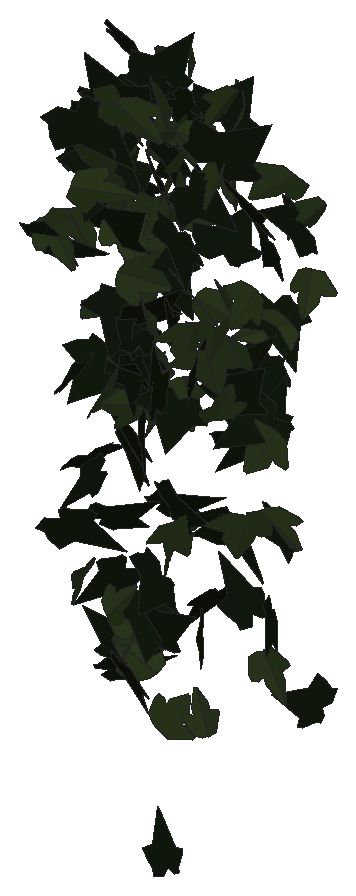
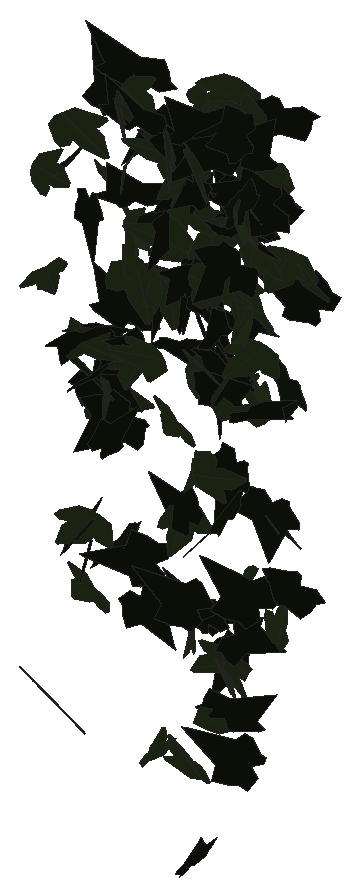
# SketchUp Ruby script. Lengths in inches.
U = 1.inch
M = Sketchup.active_model
def pt(a) = Geom::Point3d.new(a.map { |v| v * U })
def face(e, loops, mat)
  f = e.add_face(loops[0].map { |a| pt(a) })
  loops[1..].each { |l| e.add_face(l.map { |a| pt(a) }).erase! }
  f.material = f.back_material = mat if mat
  f
end
# faces: each face lists its corners as indices into pts; further lists are holes
def faces(e, pts, list, mat = nil) = list.each { |f| face(e, (f[0].is_a?(Array) ? f : [f]).map { |l| l.map { |i| pts[i] } }, mat) }
# xy, xz, yz: faces in a plane at the given z, y or x. An outline is a flat list of corners, or four numbers for a rectangle; further outlines are holes
def ring(l) = l.size == 4 ? [[l[0], l[1]], [l[2], l[1]], [l[2], l[3]], [l[0], l[3]]] : l.each_slice(2).to_a
def flat(e, list, mat, &to3) = list.each { |f| face(e, (f[0].is_a?(Array) ? f : [f]).map { |l| ring(l).map { |u, v| to3.(u, v) } }, mat) }
def xy(e, z, list, mat = nil) = flat(e, list, mat) { |x, y| [x, y, z] }
def xz(e, y, list, mat = nil) = flat(e, list, mat) { |x, z| [x, y, z] }
def yz(e, x, list, mat = nil) = flat(e, list, mat) { |y, z| [x, y, z] }
def lines(e, pts, list) = list.each { |a, b| e.add_line(pt(pts[a]), pt(pts[b])) }
# prism: a flat outline (further loops are holes) pulled along v
def prism(e, loops, v, mat = nil)
  f = face(e, loops, mat); d = Geom::Vector3d.new(v.map { |x| x * U })
  f.pushpull(f.normal.samedirection?(d) ? d.length : -d.length)
end
def box(e, o, s, mat = nil) = prism(e, [[o, [o[0] + s[0], o[1], o[2]], [o[0] + s[0], o[1] + s[1], o[2]], [o[0], o[1] + s[1], o[2]]]], [0, 0, s[2]], mat)
def at(x, y, z, deg = 0) = Geom::Transformation.translation(pt([x, y, z])) * Geom::Transformation.rotation(ORIGIN, Z_AXIS, deg.degrees)
def axes(o, x, y, z) = Geom::Transformation.new([*x, 0, *y, 0, *z, 0, *pt(o).to_a, 1])
def part(name) = M.definitions.add(name)
# library, detail: a bought-in or finely detailed component or shape, given as its bounding box
def library(name, o, s) = part(name).tap { |d| box(d.entities, o, s) }
def detail(e, o, s) = box(e.add_group.entities, o, s)
def put(e, d, t, mat = nil) = e.add_instance(d, t).tap { |i| i.material = mat if mat }
def group(e, t, mat = nil) = e.add_group.tap { |g| g.transformation = t; g.material = mat if mat }.entities
root = M.entities
M.materials.add("1026 AP 7946 SUNNY SIDE UP").color = [254, 231, 186]
M.materials.add("efeu1").color = [18, 25, 13]
M.materials.add("efeu2").color = [43, 57, 29]
c1 = part("ivyleaf_9")
p = [[1.54,2.16,1.25],[1.36,2.04,1.19],[-0.21,0.99,0.68],[-0.71,1.11,0.82],[-0.85,0.86,0.67],[-0.8,0.17,0.21],
  [-0.9,-0.01,0.1],[-0.67,-0.16,-0.02],[-0.08,-0.08,-0.05],[-0.03,-0.6,-0.4],[0.65,-0.88,-0.66],[0.83,-0.6,-0.49],
  [1.29,-0.42,-0.43],[1.8125,-0.07,-0.26],[1.21,0.44,0.15]]
faces(c1.entities,p,[[0,1,2,3,4,5,6,7,8,9,10,11,12,13,14]],"efeu1")
c2 = part("ivyleaf_10")
p = [[0,0.5,-0.03],[-0.0625,2.02,-0.43],[-0.19,2.01,-0.46],[-0.54,1.05,-0.29],[-0.52,0.625,-0.18],[-0.83,0.76,-0.28],
  [-1.16,0.64,-0.33],[-1.15,0.33,-0.24],[-0.77,-0.39,0.02],[-0.3,-0.51,0.16],[0.04,-0.48,0.23],[-0.02,2.01,-0.4375],
  [-0.06,2.01,-0.43],[0.04,-0.49,0.23],[0.67,-0.49,0.14],[1.38,0.36,-0.2],[1.375,0.51,-0.24],[0.81,0.65,-0.19],
  [0.62,0.59,-0.15],[0.6,1.09,-0.28],[0.5,1.23,-0.31]]
faces(c2.entities,p,[[0,1,2,3,4,5,6,7,8,9,10],[11,12,0,13,14,15,16,17,18,19,20]],"efeu2")
put(root,c1,axes([125.78,210.73,264.48],[0.12054,-0.07368,0.29819],[0.41686,-0.12179,-0.10483],[0.21772,0.27399,0.03562]),"1026 AP 7946 SUNNY SIDE UP")
put(root,c2,axes([125.89,211.97,264.9],[0.21507,-0.0579,0.27799],[0.37543,-0.12696,-0.1533],[0.21867,0.27492,-0.01023]),"1026 AP 7946 SUNNY SIDE UP")
put(root,c2,axes([125.91,210.6875,264.84],[0.3343,-0.00107,0.26157],[0.3907,-0.06728,-0.21503],[0.08218,0.32426,-0.04177]),"1026 AP 7946 SUNNY SIDE UP")
put(root,c1,axes([126.02,210.89,259.3],[0.02192,-0.00071,-0.30597],[0.18849,0.27204,0.00672],[0.42727,-0.11997,0.01273]),"1026 AP 7946 SUNNY SIDE UP")
put(root,c2,axes([126.32,211.97,266.5],[0.11014,-0.2742,0.11862],[0.03145,-0.11528,-0.29209],[0.46752,0.07235,-0.0083]),"1026 AP 7946 SUNNY SIDE UP")
put(root,c2,axes([126.66,212.47,261.83],[-0.1517,0.03049,-0.28411],[-0.41399,0.08267,0.10472],[0.13855,0.2804,0.00182]),"1026 AP 7946 SUNNY SIDE UP")
put(root,c2,axes([126.29,211.89,264.6],[-0.28844,0.25395,-0.1145],[0.07835,-0.10265,-0.32276],[-0.42971,-0.18918,0.018]),"1026 AP 7946 SUNNY SIDE UP")
put(root,c2,axes([126.35,210.76,265.17],[-0.42324,-0.12548,-0.09661],[0.15222,0.01154,-0.30441],[0.19279,-0.28457,0.02827]),"1026 AP 7946 SUNNY SIDE UP")
put(root,c2,axes([126.375,210.97,258.3125],[-0.02671,-0.17761,-0.27305],[-0.00878,-0.26421,0.18191],[-0.50029,0.01412,0.01138]),"1026 AP 7946 SUNNY SIDE UP")
put(root,c1,axes([126.51,210.95,260.67],[0.10897,0.30312,0.00846],[0.01022,0.00517,-0.32026],[-0.47663,0.06941,-0.00494]),"1026 AP 7946 SUNNY SIDE UP")
put(root,c2,axes([126.23,211.7,265.76],[0.4966,-0.0822,0.15346],[0.21456,-0.06688,-0.33539],[0.16088,0.34293,-0.02642]),"1026 AP 7946 SUNNY SIDE UP")
put(root,c1,axes([125.98,211.66,266.73],[0.19799,0.05636,-0.34035],[0.41951,0.19731,0.14045],[0.31977,-0.29374,0.02648]),"1026 AP 7946 SUNNY SIDE UP")
put(root,c1,axes([126.21,212.02,266.68],[0.15385,-0.20438,0.19255],[0.10869,-0.17521,-0.23423],[0.42299,0.11936,-0.00985]),"1026 AP 7946 SUNNY SIDE UP")
put(root,c2,axes([126.52,211.8,265.09],[-0.09459,-0.29834,-0.04622],[0.03148,0.03997,-0.31307],[0.47295,-0.06233,0.01159]),"1026 AP 7946 SUNNY SIDE UP")
put(root,c1,axes([126.39,211.0625,265.95],[-0.09339,0.0031,0.37339],[0.51727,0.15462,0.05508],[-0.23921,0.33313,-0.02667]),"1026 AP 7946 SUNNY SIDE UP")
put(root,c1,axes([126.33,211.59,259.15],[0.37331,0.18571,-0.05497],[0.03981,0.05558,0.30953],[0.30168,-0.23715,0.02718]),"1026 AP 7946 SUNNY SIDE UP")
put(root,c1,axes([126.28,211.96,267.99],[0.39241,-0.15583,0.11286],[0.12773,-0.07786,-0.30274],[0.27181,0.26156,-0.02067]),"1026 AP 7946 SUNNY SIDE UP")
put(root,c1,axes([126.86,211.67,265.96],[-0.47227,-0.05249,0.03408],[-0.04285,-0.03694,-0.31264],[0.08794,-0.29993,0.03071]),"1026 AP 7946 SUNNY SIDE UP")
put(root,c1,axes([126.77,210.16,262.53],[0.0099,0.23389,0.19022],[0.01171,0.18318,-0.23995],[-0.46712,0.00955,-0.00198]),"1026 AP 7946 SUNNY SIDE UP")
put(root,c1,axes([126.36,211.74,256.27],[0.27108,0.225,-0.11548],[0.08344,0.10187,0.29199],[0.38728,-0.17944,0.01792]),"1026 AP 7946 SUNNY SIDE UP")
put(root,c2,axes([126.39,211.65,266.43],[0.28057,-0.07256,0.24354],[0.34143,-0.09458,-0.19895],[0.18735,0.28102,-0.00214]),"1026 AP 7946 SUNNY SIDE UP")
put(root,c1,axes([126.92,211.57,256.87],[0.10544,0.03542,0.28985],[-0.44207,0.04453,0.06356],[-0.05584,-0.28559,0.04412]),"1026 AP 7946 SUNNY SIDE UP")
put(root,c1,axes([126.84,211.375,267.16],[0.25958,-0.00539,0.2712],[-0.39634,0.08672,0.16516],[-0.11986,-0.29841,0.0412]),"1026 AP 7946 SUNNY SIDE UP")
put(root,c1,axes([126.76,211.16,262.41],[-0.30762,-0.23846,0.12596],[-0.09814,-0.1084,-0.31779],[0.41079,-0.20447,0.01841]),"1026 AP 7946 SUNNY SIDE UP")
put(root,c1,axes([126.83,210.79,260.53],[-0.37257,0.13849,-0.12506],[0.14588,-0.08259,-0.28228],[-0.25109,-0.25348,0.02157]),"1026 AP 7946 SUNNY SIDE UP")
put(root,c1,axes([126.51,211.81,265.45],[0.45887,0.08022,0.00252],[0.01414,-0.02522,-0.31073],[-0.12539,0.29075,-0.0258]),"1026 AP 7946 SUNNY SIDE UP")
put(root,c1,axes([126.8,211.47,258.39],[-0.0435,0.00077,-0.31404],[0.10414,-0.29877,-0.00871],[-0.46789,-0.06657,0.02726]),"1026 AP 7946 SUNNY SIDE UP")
put(root,c2,axes([126.65,211.13,263.5],[-0.30292,-0.13622,-0.19501],[0.2703,0.0815,-0.24116],[0.24635,-0.25692,0.02482]),"1026 AP 7946 SUNNY SIDE UP")
put(root,c2,axes([127.2,211.83,264.95],[0.06842,-0.05078,-0.34035],[-0.48838,0.1162,-0.05992],[0.19302,0.31201,-0.03095]),"1026 AP 7946 SUNNY SIDE UP")
put(root,c2,axes([126.83,211.18,266.37],[0.07883,-0.13746,-0.3173],[0.10388,0.30859,-0.12933],[0.51893,-0.04089,0.07409]),"1026 AP 7946 SUNNY SIDE UP")
put(root,c2,axes([127,212.41,267.49],[0.22525,-0.20264,-0.1724],[-0.15575,0.13349,-0.25485],[0.38152,0.17413,-0.00225]),"1026 AP 7946 SUNNY SIDE UP")
put(root,c2,axes([126.93,212.12,261.76],[-0.02544,0.07802,0.28794],[-0.11575,0.26921,-0.08036],[-0.44066,-0.07522,0.00449]),"1026 AP 7946 SUNNY SIDE UP")
put(root,c1,axes([127.04,210.83,266.33],[-0.46572,-0.14302,-0.10495],[0.16211,0.0181,-0.33757],[0.22259,-0.31243,0.02627]),"1026 AP 7946 SUNNY SIDE UP")
put(root,c1,axes([126.88,211.78,267.5],[0.04828,-0.09551,-0.32711],[-0.00535,0.31823,-0.09726],[0.52053,0.01213,0.02934]),"1026 AP 7946 SUNNY SIDE UP")
put(root,c2,axes([127.21,211.58,256.69],[0.14116,0.22597,0.18684],[-0.1242,-0.1622,0.2493],[0.43704,-0.11908,0.0105]),"1026 AP 7946 SUNNY SIDE UP")
put(root,c1,axes([127.07,211.1875,261.32],[0.41086,-0.07086,-0.19853],[-0.30161,0.02519,-0.27791],[0.1135,0.32345,-0.01985]),"1026 AP 7946 SUNNY SIDE UP")
put(root,c1,axes([126.9,211.6,260.58],[0.05064,-0.2068,0.26901],[0.03786,-0.26139,-0.21688],[0.52384,0.03888,-0.01033]),"1026 AP 7946 SUNNY SIDE UP")
put(root,c1,axes([126.88,210.22,267.49],[-0.03588,-0.17005,-0.34523],[0.11108,0.32681,-0.1744],[0.57897,-0.07324,0.01207]),"1026 AP 7946 SUNNY SIDE UP")
put(root,c2,axes([127,210.63,266.33],[-0.47085,0.04161,0.15361],[0.22623,-0.04361,0.31045],[0.08885,0.33155,0.02356]),"1026 AP 7946 SUNNY SIDE UP")
put(root,c2,axes([127.28,211.27,257.68],[0.36603,-0.15599,-0.12256],[-0.1751,0.04526,-0.28748],[0.25294,0.25707,-0.02165]),"1026 AP 7946 SUNNY SIDE UP")
put(root,c2,axes([127.09,210.47,262.01],[0.08446,-0.3233,0.06138],[0.00964,0.0632,0.33759],[-0.51736,-0.0516,0.01631]),"1026 AP 7946 SUNNY SIDE UP")
put(root,c2,axes([127.25,212.04,258.61],[0.06787,-0.09362,-0.28402],[-0.02792,0.27681,-0.09828],[0.45617,0.03087,0.03624]),"1026 AP 7946 SUNNY SIDE UP")
put(root,c2,axes([127.22,211.33,257.59],[0.21684,-0.268,0.05727],[0.02122,-0.05722,-0.3105],[0.43034,0.13786,-0.01355]),"1026 AP 7946 SUNNY SIDE UP")
put(root,c1,axes([126.93,212.41,259.26],[0.33829,0.1653,-0.11727],[0.12075,0.08787,0.27918],[0.29249,-0.22746,0.02038]),"1026 AP 7946 SUNNY SIDE UP")
put(root,c2,axes([127.01,210.1875,266.18],[-0.09009,-0.0604,-0.33327],[0.41456,0.18752,-0.08316],[0.30881,-0.26935,0.01442]),"1026 AP 7946 SUNNY SIDE UP")
put(root,c2,axes([127,210.75,267.48],[-0.01121,0.00671,0.30978],[0.46548,0.05313,0.00632],[-0.08329,0.29601,-0.00637]),"1026 AP 7946 SUNNY SIDE UP")
put(root,c1,axes([127.36,210.85,263.82],[-0.38644,-0.14512,-0.11439],[0.17716,0.02443,-0.29181],[0.2252,-0.26823,0.03327]),"1026 AP 7946 SUNNY SIDE UP")
put(root,c2,axes([127.06,211.27,257.74],[0.24236,0.11274,0.24332],[0.33344,0.10558,-0.19439],[-0.23962,0.26094,-0.02441]),"1026 AP 7946 SUNNY SIDE UP")
put(root,c2,axes([127.45,212.43,267.64],[0.16323,-0.25345,-0.22182],[-0.05739,0.21402,-0.27827],[0.51829,0.10352,0.03904]),"1026 AP 7946 SUNNY SIDE UP")
put(root,c1,axes([127.26,211.75,267.58],[-0.19038,-0.06596,0.30627],[0.4351,0.1107,0.14187],[-0.20128,0.30168,0.01699]),"1026 AP 7946 SUNNY SIDE UP")
put(root,c2,axes([127.4375,211.56,264.52],[-0.05623,0.17635,0.30673],[0.07887,-0.29251,0.1836],[0.53701,0.06142,0.00515]),"1026 AP 7946 SUNNY SIDE UP")
put(root,c1,axes([127.26,210.57,265.31],[-0.17127,-0.01633,0.33508],[0.35546,-0.2508,0.06353],[0.36881,0.23413,0.09437]),"1026 AP 7946 SUNNY SIDE UP")
put(root,c1,axes([127.36,211.8,266.72],[0.4604,-0.08452,-0.03393],[-0.0618,-0.01967,-0.31258],[0.12824,0.29394,-0.02881]),"1026 AP 7946 SUNNY SIDE UP")
put(root,c2,axes([127.62,210.77,262.1],[-0.01517,0.12729,0.35315],[0.06368,-0.33971,0.12942],[0.57037,0.04131,-0.00506]),"1026 AP 7946 SUNNY SIDE UP")
put(root,c2,axes([127.45,210.7,265.375],[0.34569,0.22665,0.06981],[0.09908,0.03125,-0.32424],[-0.35793,0.22754,-0.02233]),"1026 AP 7946 SUNNY SIDE UP")
put(root,c2,axes([127.68,211.75,266.59],[0.04346,-0.00753,0.34432],[-0.12245,0.32604,0.01611],[-0.51129,-0.07872,0.02541]),"1026 AP 7946 SUNNY SIDE UP")
put(root,c2,axes([127.61,210.17,258.52],[0.05115,0.06951,-0.28899],[0.12448,0.26976,0.07979],[0.43767,-0.08485,0.01108]),"1026 AP 7946 SUNNY SIDE UP")
put(root,c1,axes([127.5,210.91,262.9],[-0.23222,-0.1177,-0.23213],[0.34677,0.06879,-0.18608],[0.19695,-0.25991,0.05393]),"1026 AP 7946 SUNNY SIDE UP")
put(root,c1,axes([127.53,210.9,262.33],[0.4637,-0.16133,0.01077],[0.00886,0.03388,0.34488],[-0.25415,-0.29317,0.03167]),"1026 AP 7946 SUNNY SIDE UP")
put(root,c1,axes([127.72,210.74,263.3],[-0.17694,-0.1372,0.29466],[0.25094,0.23875,0.18356],[-0.43236,0.19472,-0.01405]),"1026 AP 7946 SUNNY SIDE UP")
put(root,c2,axes([127.64,211.34,266.97],[-0.04865,-0.1505,-0.2973],[0.13835,0.27433,-0.15596],[0.49147,-0.09212,0.01448]),"1026 AP 7946 SUNNY SIDE UP")
put(root,c2,axes([127.66,211.42,266.58],[0.0542,-0.15422,0.28276],[-0.02385,0.27586,0.16274],[-0.49567,-0.03013,0.02309]),"1026 AP 7946 SUNNY SIDE UP")
put(root,c2,axes([127.5,211.6875,255.72],[0.4124,-0.11776,-0.11906],[0.18791,-0.01228,0.2939],[-0.17783,-0.28608,0.03444]),"1026 AP 7946 SUNNY SIDE UP")
put(root,c1,axes([127.64,210.4375,257.33],[0.40702,-0.08305,-0.14542],[-0.22483,0.01234,-0.27846],[0.12426,0.29436,-0.02749]),"1026 AP 7946 SUNNY SIDE UP")
put(root,c2,axes([127.74,211.19,267.79],[-0.31106,0.24008,-0.04286],[0.0176,-0.04633,-0.32004],[-0.38309,-0.19706,0.02009]),"1026 AP 7946 SUNNY SIDE UP")
put(root,c2,axes([127.61,210.49,267.73],[-0.40289,-0.10803,-0.2028],[0.3028,0.0461,-0.2849],[0.17995,-0.31944,0.02535]),"1026 AP 7946 SUNNY SIDE UP")
put(root,c1,axes([127.66,210.66,262.88],[-0.2204,-0.02321,-0.25732],[0.38941,-0.05748,-0.13808],[-0.06156,-0.28048,0.04787]),"1026 AP 7946 SUNNY SIDE UP")
put(root,c1,axes([127.8,211.6875,266.3125],[-0.0628,-0.12049,0.28843],[-0.13206,-0.26781,-0.13232],[0.46175,-0.09298,0.00139]),"1026 AP 7946 SUNNY SIDE UP")
put(root,c1,axes([127.83,210.97,258.29],[-0.32284,-0.19926,-0.11114],[0.14601,0.05714,-0.29353],[0.32408,-0.22425,0.02153]),"1026 AP 7946 SUNNY SIDE UP")
put(root,c1,axes([127.55,211.96,267.1875],[0.14626,-0.08622,-0.27948],[0.44658,0.03833,0.08815],[0.01589,-0.28375,0.09498]),"1026 AP 7946 SUNNY SIDE UP")
put(root,c1,axes([127.76,211.23,264.63],[-0.09831,-0.2241,-0.23097],[0.1208,0.20966,-0.2381],[0.48213,-0.09823,0.01256]),"1026 AP 7946 SUNNY SIDE UP")
put(root,c1,axes([128.01,211.69,265.62],[-0.00693,-0.01748,-0.30726],[-0.27088,0.24374,-0.01067],[0.38363,0.17178,-0.01309]),"1026 AP 7946 SUNNY SIDE UP")
put(root,c1,axes([127.8125,211.21,265.95],[-0.10562,0.00348,0.35669],[0.04243,-0.35155,0.00698],[0.54277,0.02816,0.06886]),"1026 AP 7946 SUNNY SIDE UP")
put(root,c1,axes([128.07,211.03,253.54],[-0.16897,-0.17454,0.21803],[0.14904,0.19081,0.21182],[-0.40607,0.14266,-0.01298]),"1026 AP 7946 SUNNY SIDE UP")
put(root,c2,axes([128.08,211.1875,265.79],[-0.09022,-0.28179,0.20872],[-0.04673,-0.20224,-0.29729],[0.5452,-0.06396,0.00906]),"1026 AP 7946 SUNNY SIDE UP")
put(root,c2,axes([128.03,210.55,264.17],[-0.17368,0.29491,0.08513],[-0.06866,0.06999,-0.32361],[-0.47595,-0.11771,0.01562]),"1026 AP 7946 SUNNY SIDE UP")
put(root,c1,axes([127.83,210.67,262.03],[-0.0862,0.00371,-0.35475],[0.48911,-0.14913,-0.05354],[-0.23243,-0.31521,0.0189]),"1026 AP 7946 SUNNY SIDE UP")
put(root,c1,axes([127.8125,210.63,263.85],[0.33208,0.23474,0.02834],[-0.05409,-0.00418,0.32443],[0.36744,-0.21277,0.02214]),"1026 AP 7946 SUNNY SIDE UP")
put(root,c2,axes([127.76,210.78,262.35],[0.10418,-0.14634,-0.26948],[0.35417,-0.15123,0.14551],[-0.30923,-0.22251,0.07587]),"1026 AP 7946 SUNNY SIDE UP")
put(root,c1,axes([127.86,211.35,266.67],[0.08987,-0.28903,0.14273],[0.04429,-0.13734,-0.30432],[0.50316,0.06371,0.00129]),"1026 AP 7946 SUNNY SIDE UP")
put(root,c2,axes([127.86,211.72,262.06],[0.36641,-0.06276,0.206],[0.28272,-0.09478,-0.24663],[0.17035,0.29231,-0.03377]),"1026 AP 7946 SUNNY SIDE UP")
put(root,c2,axes([128.02,210.15,264.875],[0.08855,0.15166,0.34153],[0.04424,0.33178,-0.15976],[-0.5703,0.04929,0.04064]),"1026 AP 7946 SUNNY SIDE UP")
put(root,c2,axes([128.14,211.26,266.59],[0.15771,-0.2863,0.18687],[0.08043,-0.17593,-0.31343],[0.52822,0.11227,-0.00807]),"1026 AP 7946 SUNNY SIDE UP")
put(root,c1,axes([128.12,211.2,263.6],[-0.01933,0.11194,0.34237],[-0.16215,-0.31834,0.10488],[0.52605,-0.09401,0.04491]),"1026 AP 7946 SUNNY SIDE UP")
put(root,c2,axes([128.23,211.8125,255.83],[0.03992,0.29255,-0.03772],[-0.01069,0.03899,0.30257],[0.46381,-0.02428,0.01022]),"1026 AP 7946 SUNNY SIDE UP")
put(root,c2,axes([127.86,211.73,265.3125],[-0.11308,-0.06976,0.2982],[0.39683,0.14451,0.10118],[-0.24959,0.26136,0.02576]),"1026 AP 7946 SUNNY SIDE UP")
put(root,c1,axes([127.94,210.82,257.96],[-0.07635,0.06909,0.29121],[0.30429,-0.20583,0.08498],[0.34092,0.19919,-0.01064]),"1026 AP 7946 SUNNY SIDE UP")
put(root,c2,axes([128.25,211.04,259.9],[-0.22236,-0.27347,-0.11429],[0.10729,0.08763,-0.31604],[0.45054,-0.15584,0.01885]),"1026 AP 7946 SUNNY SIDE UP")
put(root,c1,axes([127.95,211.3125,260.05],[0.08346,-0.05989,0.30582],[0.22973,-0.25932,-0.08223],[0.4177,0.15459,-0.01588]),"1026 AP 7946 SUNNY SIDE UP")
put(root,c2,axes([127.96,212.23,263.44],[-0.13163,-0.027,-0.29207],[0.43917,-0.06475,-0.07903],[-0.08631,-0.28828,0.04332]),"1026 AP 7946 SUNNY SIDE UP")
put(root,c2,axes([128.28,210.72,262.38],[0.0652,-0.19552,0.24021],[0.09719,-0.22615,-0.20703],[0.46987,0.07391,0.00949]),"1026 AP 7946 SUNNY SIDE UP")
put(root,c1,axes([128.29,210.57,259.19],[-0.09445,-0.2406,0.23272],[-0.07817,-0.2218,-0.25674],[0.51451,-0.07786,0.00371]),"1026 AP 7946 SUNNY SIDE UP")
put(root,c2,axes([128.08,211.625,266.87],[-0.10355,-0.03306,-0.31075],[0.45626,-0.09653,-0.05496],[-0.1386,-0.29308,0.05123]),"1026 AP 7946 SUNNY SIDE UP")
put(root,c1,axes([128.15,211.96,259.46],[0.21626,0.05833,0.26516],[0.39622,0.05602,-0.15166],[-0.12167,0.28611,-0.02255]),"1026 AP 7946 SUNNY SIDE UP")
put(root,c1,axes([128.65,210.05,262.76],[0.03278,0.03801,0.38134],[-0.03205,0.37009,-0.03582],[-0.5839,-0.01818,0.02338]),"1026 AP 7946 SUNNY SIDE UP")
put(root,c1,axes([128.61,211.65,258.51],[-0.08166,0.22363,-0.19228],[0.05124,-0.18523,-0.23746],[-0.45643,-0.06081,0.00774]),"1026 AP 7946 SUNNY SIDE UP")
put(root,c2,axes([128.6,210.78,266.24],[0.12749,-0.12778,-0.32527],[0.00105,0.3239,-0.13329],[0.53452,0.02984,0.07784]),"1026 AP 7946 SUNNY SIDE UP")
put(root,c2,axes([128.76,210.78,263.85],[-0.23402,-0.30885,0.01851],[0.01527,-0.02654,-0.35273],[0.48639,-0.14777,0.01998]),"1026 AP 7946 SUNNY SIDE UP")
put(root,c2,axes([128.78,211.74,267.81],[-0.03102,-0.25481,0.19999],[0.003,-0.19604,-0.26407],[0.50507,-0.01449,0.01385]),"1026 AP 7946 SUNNY SIDE UP")
put(root,c1,axes([128.55,210.72,265.59],[0.03695,-0.3166,0.14257],[0.02133,-0.13956,-0.32785],[0.54402,0.02697,0.00317]),"1026 AP 7946 SUNNY SIDE UP")
put(root,c1,axes([128.63,211.77,267.33],[-0.31059,0.07867,0.23355],[0.31151,-0.11121,0.21736],[0.21175,0.279,0.0228]),"1026 AP 7946 SUNNY SIDE UP")
put(root,c1,axes([128.75,210.47,262.66],[-0.30431,-0.20676,-0.06886],[0.0932,0.03426,-0.29087],[0.32813,-0.20148,0.01875]),"1026 AP 7946 SUNNY SIDE UP")
put(root,c2,axes([128.93,211.88,267.67],[0.08253,-0.15632,-0.26364],[-0.14606,0.23761,-0.16834],[0.44709,0.10648,-0.00633]),"1026 AP 7946 SUNNY SIDE UP")
put(root,c1,axes([128.91,212.27,261.5],[0.01003,0.02361,0.30827],[-0.31483,-0.22248,0.02118],[0.35136,-0.20002,0.01019]),"1026 AP 7946 SUNNY SIDE UP")
put(root,c1,axes([129.05,210.73,258.3125],[0.05433,-0.02752,-0.31487],[-0.43276,0.13291,-0.04363],[0.21289,0.27722,-0.00833]),"1026 AP 7946 SUNNY SIDE UP")
put(root,c2,axes([128.76,211.57,262.82],[0.19336,0.28483,0.0381],[0.04075,0.0273,-0.31917],[-0.44946,0.12501,-0.01255]),"1026 AP 7946 SUNNY SIDE UP")
put(root,c1,axes([128.71,211.95,259.68],[0.22765,-0.2609,-0.02659],[-0.03806,0.01436,-0.30696],[0.41026,0.14611,-0.01372]),"1026 AP 7946 SUNNY SIDE UP")
put(root,c2,axes([129.08,211.4375,266.22],[0.00125,0.1737,-0.26897],[-0.07616,0.25902,0.17822],[0.48848,0.03994,0.02847]),"1026 AP 7946 SUNNY SIDE UP")
put(root,c2,axes([129.27,212.4375,263.4],[0.25256,0.05248,-0.25874],[-0.35759,-0.10884,-0.17369],[-0.18781,0.27782,-0.01724]),"1026 AP 7946 SUNNY SIDE UP")
put(root,c1,axes([129.1875,210.39,263.53],[0.00461,-0.01618,-0.34007],[-0.38449,0.22184,-0.01215],[0.3494,0.24434,-0.00888]),"1026 AP 7946 SUNNY SIDE UP")
put(root,c1,axes([129,211.55,262.75],[-0.07174,-0.03952,0.31795],[0.40787,0.16785,0.06258],[-0.27084,0.26325,0.01003]),"1026 AP 7946 SUNNY SIDE UP")
put(root,c1,axes([129.04,210.46,266.74],[0.11242,-0.16089,-0.31414],[-0.139,0.2915,-0.17863],[0.5227,0.11212,0.02006]),"1026 AP 7946 SUNNY SIDE UP")
put(root,c1,axes([129.01,211.57,261.6875],[0.36915,0.18312,0.1027],[0.14504,0.04168,-0.30559],[-0.29315,0.25122,-0.02187]),"1026 AP 7946 SUNNY SIDE UP")
put(root,c2,axes([129.39,210.83,263.86],[-0.55432,0.01355,0.12395],[-0.19025,-0.03498,-0.36159],[-0.00231,-0.37083,0.03645]),"1026 AP 7946 SUNNY SIDE UP")
put(root,c1,axes([128.85,210.54,264.79],[0.31921,-0.24311,0.14634],[0.13253,-0.11641,-0.32683],[0.42359,0.21962,-0.00802]),"1026 AP 7946 SUNNY SIDE UP")
put(root,c1,axes([129.11,212.38,262.75],[-0.07901,-0.27899,0.10528],[-0.02409,-0.10268,-0.29263],[0.46744,-0.05245,0.00271]),"1026 AP 7946 SUNNY SIDE UP")
put(root,c2,axes([129.39,211.57,261.89],[0.02812,-0.00118,0.32406],[-0.2836,0.25811,0.01307],[-0.40526,-0.18071,0.01334]),"1026 AP 7946 SUNNY SIDE UP")
put(root,c1,axes([129.09,212.57,263.625],[-0.05331,-0.3009,-0.13692],[0.02933,0.12992,-0.31116],[0.51532,-0.03852,0.00355]),"1026 AP 7946 SUNNY SIDE UP")
put(root,c2,axes([129.27,211.19,264.23],[-0.34391,0.20997,0.11092],[0.14649,-0.05628,0.31115],[0.33996,0.23666,-0.02186]),"1026 AP 7946 SUNNY SIDE UP")
put(root,c1,axes([129.26,211.04,265.39],[-0.30162,-0.023,0.23752],[0.35614,0.04528,0.19894],[-0.07777,0.29658,-0.01017]),"1026 AP 7946 SUNNY SIDE UP")
put(root,c2,axes([129.36,210.5,263.6875],[-0.4094,-0.22396,-0.06199],[0.09731,0.01812,-0.35266],[0.35089,-0.26633,0.02547]),"1026 AP 7946 SUNNY SIDE UP")
put(root,c2,axes([129.27,212.17,259.9375],[-0.37167,-0.07888,-0.17345],[0.26494,0.02257,-0.25512],[0.1221,-0.28906,0.02559]),"1026 AP 7946 SUNNY SIDE UP")
put(root,c1,axes([129.38,212.39,259.67],[0.19473,-0.22951,-0.16125],[0.15064,-0.12406,0.267],[-0.40879,-0.15505,0.02157]),"1026 AP 7946 SUNNY SIDE UP")
put(root,c1,axes([129.65,211.24,258.72],[-0.20984,-0.25089,0.14079],[0.07681,0.13017,0.29304],[-0.4437,0.14118,-0.01585]),"1026 AP 7946 SUNNY SIDE UP")
put(root,c2,axes([129.44,210.62,267.16],[0.3106,-0.23732,0.09669],[0.07512,-0.08394,-0.31815],[0.395,0.20258,-0.01553]),"1026 AP 7946 SUNNY SIDE UP")
put(root,c1,axes([129.6875,211.66,265.45],[0.23411,-0.04491,-0.28596],[-0.42855,0.05302,-0.15928],[0.10712,0.31026,-0.01226]),"1026 AP 7946 SUNNY SIDE UP")
put(root,c1,axes([129.46,210.625,267.34],[-0.24363,0.084,0.32797],[0.45469,-0.13243,0.18048],[0.24605,0.3279,-0.00877]),"1026 AP 7946 SUNNY SIDE UP")
put(root,c1,axes([129.86,211.29,262.06],[-0.02812,0.11083,-0.28943],[0.01581,-0.2817,-0.11653],[-0.47555,-0.01592,0.01324]),"1026 AP 7946 SUNNY SIDE UP")
put(root,c2,axes([129.72,210.36,262.82],[-0.15272,-0.2767,0.01564],[-0.00531,0.01893,0.30206],[-0.43585,0.09673,-0.00916]),"1026 AP 7946 SUNNY SIDE UP")
put(root,c1,axes([129.81,211.43,262.12],[-0.34357,0.22539,-0.03087],[-0.0154,0.03397,0.32314],[0.35746,0.2181,-0.01575]),"1026 AP 7946 SUNNY SIDE UP")
put(root,c2,axes([129.78,210.45,264.42],[0.1055,-0.23734,0.18478],[0.0764,-0.17405,-0.2551],[0.46279,0.08284,-0.00001]),"1026 AP 7946 SUNNY SIDE UP")
put(root,c2,axes([130.08,211.64,266.77],[-0.30341,-0.12929,0.22006],[-0.25222,-0.14391,-0.23902],[0.30217,-0.24994,0.02145]),"1026 AP 7946 SUNNY SIDE UP")
put(root,c1,axes([129.63,210.73,262.91],[-0.23586,0.01423,0.27987],[0.36327,-0.15697,0.139],[0.22562,0.26762,0.06876]),"1026 AP 7946 SUNNY SIDE UP")
put(root,c1,axes([130.21,212.34,256.66],[-0.26493,0.21018,0.15333],[-0.16664,0.10395,-0.27644],[-0.36789,-0.19844,0.0148]),"1026 AP 7946 SUNNY SIDE UP")
put(root,c2,axes([129.91,212.48,264.47],[0.17414,0.25912,-0.11788],[-0.05398,-0.11126,-0.29072],[-0.44305,0.1154,-0.01091]),"1026 AP 7946 SUNNY SIDE UP")
put(root,c1,axes([130.24,211.04,262.62],[-0.41153,-0.14117,0.1123],[-0.13117,-0.07582,-0.30566],[0.24876,-0.27351,0.02462]),"1026 AP 7946 SUNNY SIDE UP")
put(root,c1,axes([129.95,211.41,258.7],[0.06666,-0.08027,-0.316],[0.38972,-0.18388,0.08391],[-0.30982,-0.24858,0.03756]),"1026 AP 7946 SUNNY SIDE UP")
put(root,c2,axes([130.3,210.3,261.02],[-0.34122,-0.26673,0.0492],[-0.02184,-0.05208,-0.35382],[0.42594,-0.21634,0.02127]),"1026 AP 7946 SUNNY SIDE UP")
put(root,c1,axes([130.26,211.83,265.86],[0.1285,-0.29748,-0.10159],[0.05797,-0.09032,0.31708],[-0.48853,-0.08897,0.01091]),"1026 AP 7946 SUNNY SIDE UP")
put(root,c2,axes([130.28,212.14,266.06],[-0.0094,-0.18941,0.24263],[0.00459,-0.23667,-0.1965],[0.47653,-0.00146,0.00668]),"1026 AP 7946 SUNNY SIDE UP")
put(root,c2,axes([130.3,210.39,265.18],[0.40921,-0.18661,-0.04904],[-0.07749,0.011,-0.32922],[0.29231,0.26414,-0.01862]),"1026 AP 7946 SUNNY SIDE UP")
put(root,c2,axes([130.04,211.15,257.97],[0.3419,-0.03509,0.23027],[0.33932,-0.06189,-0.22644],[0.10792,0.30577,-0.01753]),"1026 AP 7946 SUNNY SIDE UP")
put(root,c2,axes([130.38,210.78,262.4],[0.49855,-0.12436,-0.06978],[-0.11232,0.00096,-0.34993],[0.19164,0.32407,-0.02357]),"1026 AP 7946 SUNNY SIDE UP")
put(root,c1,axes([130.04,210.49,266.84],[0.42275,-0.10488,-0.20001],[0.29602,-0.04884,0.29637],[-0.17944,-0.32766,0.01769]),"1026 AP 7946 SUNNY SIDE UP")
